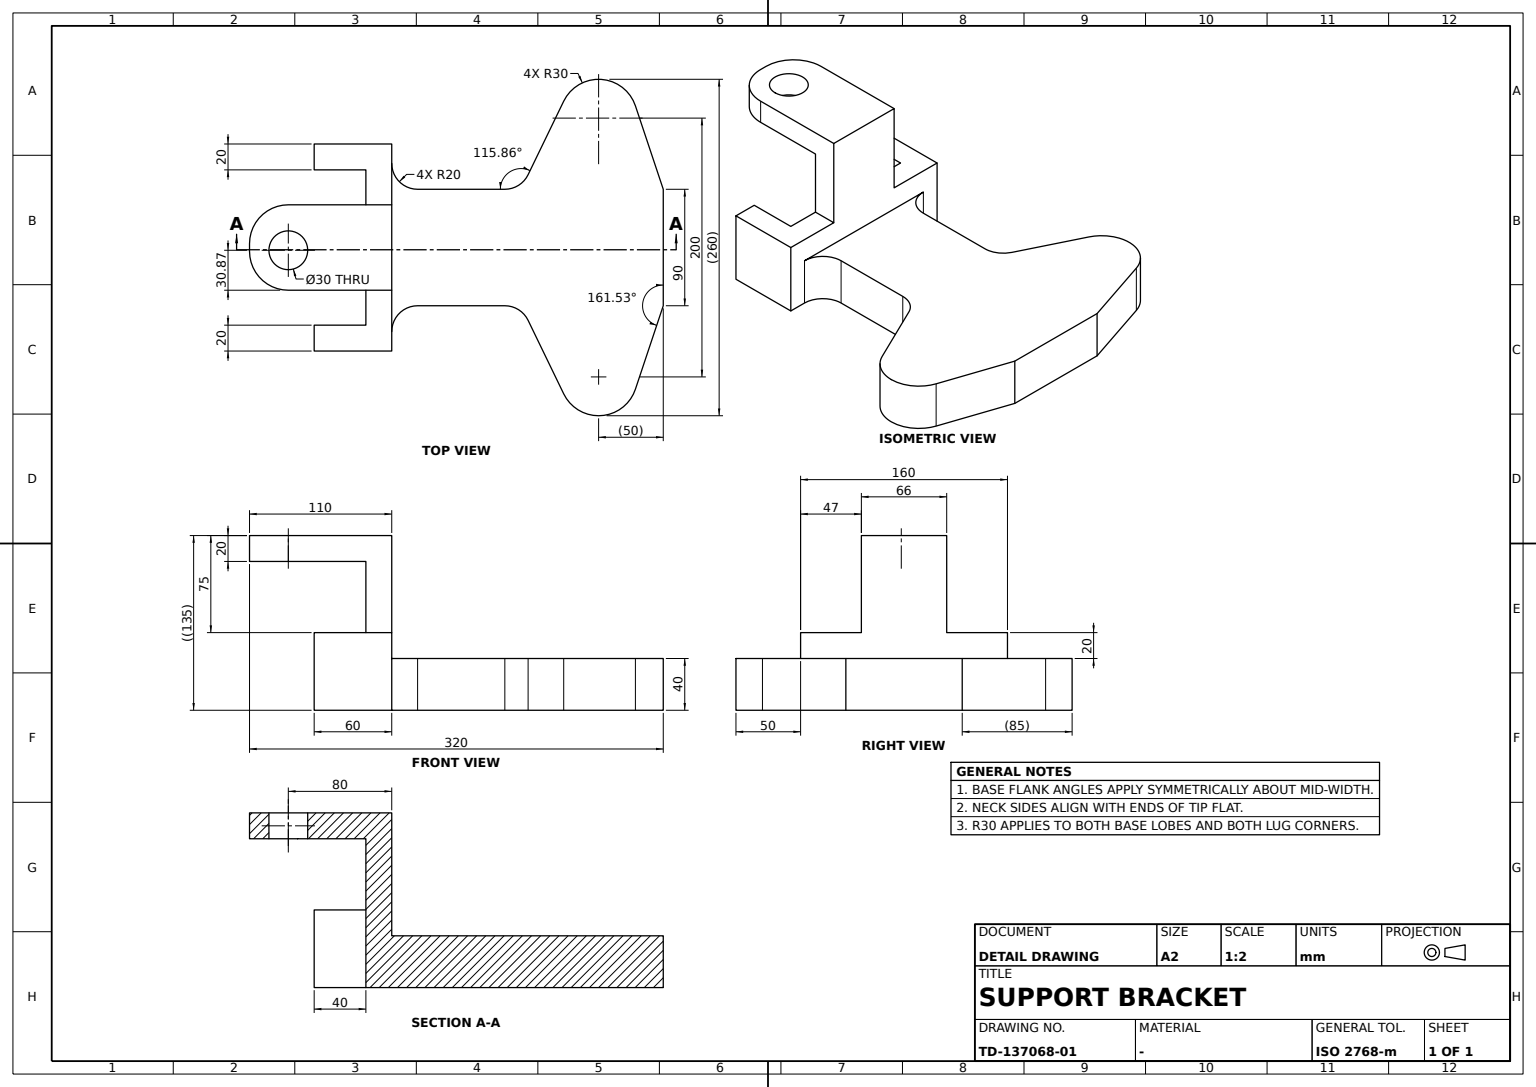
ISO-10303-21;
HEADER;
FILE_DESCRIPTION((''),'2;1');
FILE_NAME('','',(''),(''),'','','');
FILE_SCHEMA(('AUTOMOTIVE_DESIGN'));
ENDSEC;
DATA;
#1=APPLICATION_CONTEXT('');
#2=PRODUCT_CONTEXT('',#1,'mechanical');
#3=PRODUCT('','','',(#2));
#4=PRODUCT_DEFINITION_FORMATION('','',#3);
#5=PRODUCT_DEFINITION_CONTEXT('',#1,'design');
#6=PRODUCT_DEFINITION('','',#4,#5);
#7=PRODUCT_DEFINITION_SHAPE('','',#6);
#8=(LENGTH_UNIT()NAMED_UNIT(*)SI_UNIT(.MILLI.,.METRE.));
#9=(NAMED_UNIT(*)PLANE_ANGLE_UNIT()SI_UNIT($,.RADIAN.));
#10=(NAMED_UNIT(*)SI_UNIT($,.STERADIAN.)SOLID_ANGLE_UNIT());
#11=UNCERTAINTY_MEASURE_WITH_UNIT(LENGTH_MEASURE(1.E-05),#8,'distance_accuracy_value','');
#12=(GEOMETRIC_REPRESENTATION_CONTEXT(3)GLOBAL_UNCERTAINTY_ASSIGNED_CONTEXT((#11))GLOBAL_UNIT_ASSIGNED_CONTEXT((#8,#9,#10))REPRESENTATION_CONTEXT('',''));
#13=CARTESIAN_POINT('',(-80.,-220.,0.));
#14=VERTEX_POINT('',#13);
#15=CARTESIAN_POINT('',(-80.,-220.,60.));
#16=VERTEX_POINT('',#15);
#17=CARTESIAN_POINT('',(-80.,-220.,30.));
#18=DIRECTION('',(0.,0.,1.));
#19=VECTOR('',#18,1000.);
#20=LINE('',#17,#19);
#21=EDGE_CURVE('',#14,#16,#20,.T.);
#22=ORIENTED_EDGE('',*,*,#21,.T.);
#23=CARTESIAN_POINT('',(-80.,-160.,60.));
#24=VERTEX_POINT('',#23);
#25=CARTESIAN_POINT('',(-80.,-190.,60.));
#26=DIRECTION('',(0.,1.,0.));
#27=VECTOR('',#26,1000.);
#28=LINE('',#25,#27);
#29=EDGE_CURVE('',#16,#24,#28,.T.);
#30=ORIENTED_EDGE('',*,*,#29,.T.);
#31=CARTESIAN_POINT('',(-80.,-160.,0.));
#32=VERTEX_POINT('',#31);
#33=CARTESIAN_POINT('',(-80.,-160.,30.));
#34=LINE('',#33,#19);
#35=EDGE_CURVE('',#32,#24,#34,.T.);
#36=ORIENTED_EDGE('',*,*,#35,.F.);
#37=CARTESIAN_POINT('',(-80.,-190.,0.));
#38=LINE('',#37,#27);
#39=EDGE_CURVE('',#14,#32,#38,.T.);
#40=ORIENTED_EDGE('',*,*,#39,.F.);
#41=EDGE_LOOP('',(#22,#30,#36,#40));
#42=FACE_OUTER_BOUND('',#41,.T.);
#43=DIRECTION('',(-1.,0.,0.));
#44=DIRECTION('',(0.,-1.,0.));
#45=AXIS2_PLACEMENT_3D('',#31,#43,#44);
#46=PLANE('',#45);
#47=ADVANCED_FACE('',(#42),#46,.T.);
#48=CARTESIAN_POINT('',(33.,-240.,135.));
#49=VERTEX_POINT('',#48);
#50=CARTESIAN_POINT('',(33.,-240.,115.));
#51=VERTEX_POINT('',#50);
#52=CARTESIAN_POINT('',(33.,-240.,125.));
#53=DIRECTION('',(0.,0.,-1.));
#54=VECTOR('',#53,1000.);
#55=LINE('',#52,#54);
#56=EDGE_CURVE('',#49,#51,#55,.T.);
#57=ORIENTED_EDGE('',*,*,#56,.F.);
#58=CARTESIAN_POINT('',(3.,-270.,135.));
#59=VERTEX_POINT('',#58);
#60=CARTESIAN_POINT('',(3.,-240.,135.));
#61=AXIS2_PLACEMENT_3D('',#60,#53,#44);
#62=CIRCLE('',#61,30.);
#63=EDGE_CURVE('',#49,#59,#62,.T.);
#64=ORIENTED_EDGE('',*,*,#63,.T.);
#65=CARTESIAN_POINT('',(3.,-270.,115.));
#66=VERTEX_POINT('',#65);
#67=CARTESIAN_POINT('',(3.,-270.,125.));
#68=LINE('',#67,#54);
#69=EDGE_CURVE('',#59,#66,#68,.T.);
#70=ORIENTED_EDGE('',*,*,#69,.T.);
#71=CARTESIAN_POINT('',(3.,-240.,115.));
#72=AXIS2_PLACEMENT_3D('',#71,#18,#44);
#73=CIRCLE('',#72,30.);
#74=EDGE_CURVE('',#66,#51,#73,.T.);
#75=ORIENTED_EDGE('',*,*,#74,.T.);
#76=EDGE_LOOP('',(#57,#64,#70,#75));
#77=FACE_OUTER_BOUND('',#76,.T.);
#78=CARTESIAN_POINT('',(3.,-240.,97.5));
#79=AXIS2_PLACEMENT_3D('',#78,#18,#44);
#80=CYLINDRICAL_SURFACE('',#79,30.);
#81=ADVANCED_FACE('',(#77),#80,.T.);
#82=CARTESIAN_POINT('',(-56.276004,-54.533987,0.));
#83=VERTEX_POINT('',#82);
#84=CARTESIAN_POINT('',(-45.,-72.530984,0.));
#85=VERTEX_POINT('',#84);
#86=CARTESIAN_POINT('',(-65.,-72.530984,0.));
#87=DIRECTION('',(1.,0.,0.));
#88=AXIS2_PLACEMENT_3D('',#86,#53,#87);
#89=CIRCLE('',#88,20.);
#90=EDGE_CURVE('',#83,#85,#89,.T.);
#91=ORIENTED_EDGE('',*,*,#90,.T.);
#92=CARTESIAN_POINT('',(-45.,-72.530984,40.));
#93=VERTEX_POINT('',#92);
#94=CARTESIAN_POINT('',(-45.,-72.530984,20.));
#95=LINE('',#94,#19);
#96=EDGE_CURVE('',#85,#93,#95,.T.);
#97=ORIENTED_EDGE('',*,*,#96,.T.);
#98=CARTESIAN_POINT('',(-56.276004,-54.533987,40.));
#99=VERTEX_POINT('',#98);
#100=CARTESIAN_POINT('',(-65.,-72.530984,40.));
#101=AXIS2_PLACEMENT_3D('',#100,#53,#87);
#102=CIRCLE('',#101,20.);
#103=EDGE_CURVE('',#99,#93,#102,.T.);
#104=ORIENTED_EDGE('',*,*,#103,.F.);
#105=CARTESIAN_POINT('',(-56.276004,-54.533987,20.));
#106=LINE('',#105,#19);
#107=EDGE_CURVE('',#83,#99,#106,.T.);
#108=ORIENTED_EDGE('',*,*,#107,.F.);
#109=EDGE_LOOP('',(#91,#97,#104,#108));
#110=FACE_OUTER_BOUND('',#109,.T.);
#111=CARTESIAN_POINT('',(-65.,-72.530984,10.));
#112=AXIS2_PLACEMENT_3D('',#111,#53,#87);
#113=CYLINDRICAL_SURFACE('',#112,20.);
#114=ADVANCED_FACE('',(#110),#113,.F.);
#115=CARTESIAN_POINT('',(-109.504259,28.454684,0.));
#116=VERTEX_POINT('',#115);
#117=CARTESIAN_POINT('',(-109.504259,28.454684,40.));
#118=VERTEX_POINT('',#117);
#119=CARTESIAN_POINT('',(-109.504259,28.454684,20.));
#120=LINE('',#119,#19);
#121=EDGE_CURVE('',#116,#118,#120,.T.);
#122=ORIENTED_EDGE('',*,*,#121,.F.);
#123=CARTESIAN_POINT('',(-113.085994,-26.995495,0.));
#124=VERTEX_POINT('',#123);
#125=CARTESIAN_POINT('',(-100.,0.,0.));
#126=AXIS2_PLACEMENT_3D('',#125,#18,#87);
#127=CIRCLE('',#126,30.);
#128=EDGE_CURVE('',#116,#124,#127,.T.);
#129=ORIENTED_EDGE('',*,*,#128,.T.);
#130=CARTESIAN_POINT('',(-113.085994,-26.995495,40.));
#131=VERTEX_POINT('',#130);
#132=CARTESIAN_POINT('',(-113.085994,-26.995495,20.));
#133=LINE('',#132,#19);
#134=EDGE_CURVE('',#124,#131,#133,.T.);
#135=ORIENTED_EDGE('',*,*,#134,.T.);
#136=CARTESIAN_POINT('',(-100.,0.,40.));
#137=AXIS2_PLACEMENT_3D('',#136,#18,#87);
#138=CIRCLE('',#137,30.);
#139=EDGE_CURVE('',#118,#131,#138,.T.);
#140=ORIENTED_EDGE('',*,*,#139,.F.);
#141=EDGE_LOOP('',(#122,#129,#135,#140));
#142=FACE_OUTER_BOUND('',#141,.T.);
#143=CARTESIAN_POINT('',(-100.,0.,10.));
#144=AXIS2_PLACEMENT_3D('',#143,#53,#87);
#145=CYLINDRICAL_SURFACE('',#144,30.);
#146=ADVANCED_FACE('',(#142),#145,.T.);
#147=CARTESIAN_POINT('',(-33.,-160.,60.));
#148=VERTEX_POINT('',#147);
#149=CARTESIAN_POINT('',(-56.5,-160.,60.));
#150=VECTOR('',#87,1000.);
#151=LINE('',#149,#150);
#152=EDGE_CURVE('',#24,#148,#151,.T.);
#153=ORIENTED_EDGE('',*,*,#152,.F.);
#154=ORIENTED_EDGE('',*,*,#29,.F.);
#155=CARTESIAN_POINT('',(-60.,-220.,60.));
#156=VERTEX_POINT('',#155);
#157=CARTESIAN_POINT('',(-70.,-220.,60.));
#158=VECTOR('',#43,1000.);
#159=LINE('',#157,#158);
#160=EDGE_CURVE('',#156,#16,#159,.T.);
#161=ORIENTED_EDGE('',*,*,#160,.F.);
#162=CARTESIAN_POINT('',(-60.,-180.,60.));
#163=VERTEX_POINT('',#162);
#164=CARTESIAN_POINT('',(-60.,-200.,60.));
#165=VECTOR('',#44,1000.);
#166=LINE('',#164,#165);
#167=EDGE_CURVE('',#163,#156,#166,.T.);
#168=ORIENTED_EDGE('',*,*,#167,.F.);
#169=CARTESIAN_POINT('',(-33.,-180.,60.));
#170=VERTEX_POINT('',#169);
#171=CARTESIAN_POINT('',(-46.5,-180.,60.));
#172=LINE('',#171,#158);
#173=EDGE_CURVE('',#170,#163,#172,.T.);
#174=ORIENTED_EDGE('',*,*,#173,.F.);
#175=CARTESIAN_POINT('',(-33.,-170.,60.));
#176=LINE('',#175,#27);
#177=EDGE_CURVE('',#170,#148,#176,.T.);
#178=ORIENTED_EDGE('',*,*,#177,.T.);
#179=EDGE_LOOP('',(#153,#154,#161,#168,#174,#178));
#180=FACE_OUTER_BOUND('',#179,.T.);
#181=CARTESIAN_POINT('',(0.,0.,60.));
#182=AXIS2_PLACEMENT_3D('',#181,#53,#87);
#183=PLANE('',#182);
#184=ADVANCED_FACE('',(#180),#183,.F.);
#185=CARTESIAN_POINT('',(45.,50.,40.));
#186=VERTEX_POINT('',#185);
#187=CARTESIAN_POINT('',(-45.,50.,40.));
#188=VERTEX_POINT('',#187);
#189=CARTESIAN_POINT('',(0.,50.,40.));
#190=LINE('',#189,#158);
#191=EDGE_CURVE('',#186,#188,#190,.T.);
#192=ORIENTED_EDGE('',*,*,#191,.F.);
#193=CARTESIAN_POINT('',(45.,50.,0.));
#194=VERTEX_POINT('',#193);
#195=CARTESIAN_POINT('',(45.,50.,20.));
#196=LINE('',#195,#19);
#197=EDGE_CURVE('',#194,#186,#196,.T.);
#198=ORIENTED_EDGE('',*,*,#197,.F.);
#199=CARTESIAN_POINT('',(-45.,50.,0.));
#200=VERTEX_POINT('',#199);
#201=CARTESIAN_POINT('',(0.,50.,0.));
#202=LINE('',#201,#158);
#203=EDGE_CURVE('',#194,#200,#202,.T.);
#204=ORIENTED_EDGE('',*,*,#203,.T.);
#205=CARTESIAN_POINT('',(-45.,50.,20.));
#206=LINE('',#205,#19);
#207=EDGE_CURVE('',#200,#188,#206,.T.);
#208=ORIENTED_EDGE('',*,*,#207,.T.);
#209=EDGE_LOOP('',(#192,#198,#204,#208));
#210=FACE_OUTER_BOUND('',#209,.T.);
#211=AXIS2_PLACEMENT_3D('',#199,#44,#87);
#212=PLANE('',#211);
#213=ADVANCED_FACE('',(#210),#212,.F.);
#214=CARTESIAN_POINT('',(130.,0.,40.));
#215=VERTEX_POINT('',#214);
#216=CARTESIAN_POINT('',(109.504259,28.454684,40.));
#217=VERTEX_POINT('',#216);
#218=CARTESIAN_POINT('',(100.,0.,40.));
#219=AXIS2_PLACEMENT_3D('',#218,#18,#87);
#220=CIRCLE('',#219,30.);
#221=EDGE_CURVE('',#215,#217,#220,.T.);
#222=ORIENTED_EDGE('',*,*,#221,.F.);
#223=CARTESIAN_POINT('',(130.,0.,0.));
#224=VERTEX_POINT('',#223);
#225=CARTESIAN_POINT('',(130.,0.,10.));
#226=LINE('',#225,#54);
#227=EDGE_CURVE('',#215,#224,#226,.T.);
#228=ORIENTED_EDGE('',*,*,#227,.T.);
#229=CARTESIAN_POINT('',(109.504259,28.454684,0.));
#230=VERTEX_POINT('',#229);
#231=CARTESIAN_POINT('',(100.,0.,0.));
#232=AXIS2_PLACEMENT_3D('',#231,#18,#87);
#233=CIRCLE('',#232,30.);
#234=EDGE_CURVE('',#224,#230,#233,.T.);
#235=ORIENTED_EDGE('',*,*,#234,.T.);
#236=CARTESIAN_POINT('',(109.504259,28.454684,20.));
#237=LINE('',#236,#19);
#238=EDGE_CURVE('',#230,#217,#237,.T.);
#239=ORIENTED_EDGE('',*,*,#238,.T.);
#240=EDGE_LOOP('',(#222,#228,#235,#239));
#241=FACE_OUTER_BOUND('',#240,.T.);
#242=CARTESIAN_POINT('',(100.,0.,10.));
#243=AXIS2_PLACEMENT_3D('',#242,#53,#87);
#244=CYLINDRICAL_SURFACE('',#243,30.);
#245=ADVANCED_FACE('',(#241),#244,.T.);
#246=CARTESIAN_POINT('',(60.,-220.,60.));
#247=VERTEX_POINT('',#246);
#248=CARTESIAN_POINT('',(60.,-180.,60.));
#249=VERTEX_POINT('',#248);
#250=CARTESIAN_POINT('',(60.,-200.,60.));
#251=LINE('',#250,#27);
#252=EDGE_CURVE('',#247,#249,#251,.T.);
#253=ORIENTED_EDGE('',*,*,#252,.T.);
#254=CARTESIAN_POINT('',(60.,-180.,0.));
#255=VERTEX_POINT('',#254);
#256=CARTESIAN_POINT('',(60.,-180.,30.));
#257=LINE('',#256,#19);
#258=EDGE_CURVE('',#255,#249,#257,.T.);
#259=ORIENTED_EDGE('',*,*,#258,.F.);
#260=CARTESIAN_POINT('',(60.,-220.,0.));
#261=VERTEX_POINT('',#260);
#262=CARTESIAN_POINT('',(60.,-200.,0.));
#263=LINE('',#262,#27);
#264=EDGE_CURVE('',#261,#255,#263,.T.);
#265=ORIENTED_EDGE('',*,*,#264,.F.);
#266=CARTESIAN_POINT('',(60.,-220.,30.));
#267=LINE('',#266,#19);
#268=EDGE_CURVE('',#261,#247,#267,.T.);
#269=ORIENTED_EDGE('',*,*,#268,.T.);
#270=EDGE_LOOP('',(#253,#259,#265,#269));
#271=FACE_OUTER_BOUND('',#270,.T.);
#272=AXIS2_PLACEMENT_3D('',#254,#43,#44);
#273=PLANE('',#272);
#274=ADVANCED_FACE('',(#271),#273,.T.);
#275=CARTESIAN_POINT('',(15.289832,-247.191383,115.));
#276=VERTEX_POINT('',#275);
#277=CARTESIAN_POINT('',(15.289832,-247.191383,135.));
#278=VERTEX_POINT('',#277);
#279=CARTESIAN_POINT('',(15.289832,-247.191383,125.155));
#280=LINE('',#279,#19);
#281=EDGE_CURVE('',#276,#278,#280,.T.);
#282=ORIENTED_EDGE('',*,*,#281,.F.);
#283=CARTESIAN_POINT('',(-11.037645,-232.808617,115.));
#284=VERTEX_POINT('',#283);
#285=CARTESIAN_POINT('',(2.126093,-240.,115.));
#286=AXIS2_PLACEMENT_3D('',#285,#53,#87);
#287=CIRCLE('',#286,15.);
#288=EDGE_CURVE('',#276,#284,#287,.T.);
#289=ORIENTED_EDGE('',*,*,#288,.T.);
#290=CARTESIAN_POINT('',(-11.037645,-232.808617,135.));
#291=VERTEX_POINT('',#290);
#292=CARTESIAN_POINT('',(-11.037645,-232.808617,125.155));
#293=LINE('',#292,#19);
#294=EDGE_CURVE('',#284,#291,#293,.T.);
#295=ORIENTED_EDGE('',*,*,#294,.T.);
#296=CARTESIAN_POINT('',(2.126093,-240.,135.));
#297=AXIS2_PLACEMENT_3D('',#296,#18,#44);
#298=CIRCLE('',#297,15.);
#299=EDGE_CURVE('',#291,#278,#298,.T.);
#300=ORIENTED_EDGE('',*,*,#299,.T.);
#301=EDGE_LOOP('',(#282,#289,#295,#300));
#302=FACE_OUTER_BOUND('',#301,.T.);
#303=CARTESIAN_POINT('',(2.126093,-240.,134.9));
#304=AXIS2_PLACEMENT_3D('',#303,#18,#87);
#305=CYLINDRICAL_SURFACE('',#304,15.);
#306=ADVANCED_FACE('',(#302),#305,.F.);
#307=ORIENTED_EDGE('',*,*,#227,.F.);
#308=CARTESIAN_POINT('',(113.085994,-26.995495,40.));
#309=VERTEX_POINT('',#308);
#310=EDGE_CURVE('',#309,#215,#220,.T.);
#311=ORIENTED_EDGE('',*,*,#310,.F.);
#312=CARTESIAN_POINT('',(113.085994,-26.995495,0.));
#313=VERTEX_POINT('',#312);
#314=CARTESIAN_POINT('',(113.085994,-26.995495,20.));
#315=LINE('',#314,#19);
#316=EDGE_CURVE('',#313,#309,#315,.T.);
#317=ORIENTED_EDGE('',*,*,#316,.F.);
#318=EDGE_CURVE('',#313,#224,#233,.T.);
#319=ORIENTED_EDGE('',*,*,#318,.T.);
#320=EDGE_LOOP('',(#307,#311,#317,#319));
#321=FACE_OUTER_BOUND('',#320,.T.);
#322=ADVANCED_FACE('',(#321),#244,.T.);
#323=CARTESIAN_POINT('',(17.126093,-240.,135.));
#324=VERTEX_POINT('',#323);
#325=EDGE_CURVE('',#324,#291,#298,.T.);
#326=ORIENTED_EDGE('',*,*,#325,.T.);
#327=ORIENTED_EDGE('',*,*,#294,.F.);
#328=CARTESIAN_POINT('',(17.126093,-240.,115.));
#329=VERTEX_POINT('',#328);
#330=EDGE_CURVE('',#284,#329,#287,.T.);
#331=ORIENTED_EDGE('',*,*,#330,.T.);
#332=CARTESIAN_POINT('',(17.126093,-240.,134.9));
#333=LINE('',#332,#19);
#334=EDGE_CURVE('',#329,#324,#333,.T.);
#335=ORIENTED_EDGE('',*,*,#334,.T.);
#336=EDGE_LOOP('',(#326,#327,#331,#335));
#337=FACE_OUTER_BOUND('',#336,.T.);
#338=ADVANCED_FACE('',(#337),#305,.F.);
#339=CARTESIAN_POINT('',(-77.252129,39.227342,0.));
#340=DIRECTION('',(-0.948489482,-0.31680862,0.));
#341=VECTOR('',#340,1000.);
#342=LINE('',#339,#341);
#343=EDGE_CURVE('',#200,#116,#342,.T.);
#344=ORIENTED_EDGE('',*,*,#343,.T.);
#345=ORIENTED_EDGE('',*,*,#121,.T.);
#346=CARTESIAN_POINT('',(-77.252129,39.227342,40.));
#347=LINE('',#346,#341);
#348=EDGE_CURVE('',#188,#118,#347,.T.);
#349=ORIENTED_EDGE('',*,*,#348,.F.);
#350=ORIENTED_EDGE('',*,*,#207,.F.);
#351=EDGE_LOOP('',(#344,#345,#349,#350));
#352=FACE_OUTER_BOUND('',#351,.T.);
#353=DIRECTION('',(0.31680862,-0.948489482,0.));
#354=DIRECTION('',(0.948489482,0.31680862,0.));
#355=AXIS2_PLACEMENT_3D('',#115,#353,#354);
#356=PLANE('',#355);
#357=ADVANCED_FACE('',(#352),#356,.F.);
#358=CARTESIAN_POINT('',(-45.,-140.,0.));
#359=VERTEX_POINT('',#358);
#360=CARTESIAN_POINT('',(-65.,-160.,0.));
#361=VERTEX_POINT('',#360);
#362=CARTESIAN_POINT('',(-65.,-140.,0.));
#363=AXIS2_PLACEMENT_3D('',#362,#53,#87);
#364=CIRCLE('',#363,20.);
#365=EDGE_CURVE('',#359,#361,#364,.T.);
#366=ORIENTED_EDGE('',*,*,#365,.T.);
#367=CARTESIAN_POINT('',(-65.,-160.,40.));
#368=VERTEX_POINT('',#367);
#369=CARTESIAN_POINT('',(-65.,-160.,20.));
#370=LINE('',#369,#19);
#371=EDGE_CURVE('',#361,#368,#370,.T.);
#372=ORIENTED_EDGE('',*,*,#371,.T.);
#373=CARTESIAN_POINT('',(-45.,-140.,40.));
#374=VERTEX_POINT('',#373);
#375=CARTESIAN_POINT('',(-65.,-140.,40.));
#376=AXIS2_PLACEMENT_3D('',#375,#53,#87);
#377=CIRCLE('',#376,20.);
#378=EDGE_CURVE('',#374,#368,#377,.T.);
#379=ORIENTED_EDGE('',*,*,#378,.F.);
#380=CARTESIAN_POINT('',(-45.,-140.,20.));
#381=LINE('',#380,#19);
#382=EDGE_CURVE('',#359,#374,#381,.T.);
#383=ORIENTED_EDGE('',*,*,#382,.F.);
#384=EDGE_LOOP('',(#366,#372,#379,#383));
#385=FACE_OUTER_BOUND('',#384,.T.);
#386=CARTESIAN_POINT('',(-65.,-140.,10.));
#387=AXIS2_PLACEMENT_3D('',#386,#53,#87);
#388=CYLINDRICAL_SURFACE('',#387,20.);
#389=ADVANCED_FACE('',(#385),#388,.F.);
#390=ORIENTED_EDGE('',*,*,#268,.F.);
#391=CARTESIAN_POINT('',(80.,-220.,0.));
#392=VERTEX_POINT('',#391);
#393=CARTESIAN_POINT('',(70.,-220.,0.));
#394=LINE('',#393,#158);
#395=EDGE_CURVE('',#392,#261,#394,.T.);
#396=ORIENTED_EDGE('',*,*,#395,.F.);
#397=CARTESIAN_POINT('',(80.,-220.,60.));
#398=VERTEX_POINT('',#397);
#399=CARTESIAN_POINT('',(80.,-220.,30.));
#400=LINE('',#399,#19);
#401=EDGE_CURVE('',#392,#398,#400,.T.);
#402=ORIENTED_EDGE('',*,*,#401,.T.);
#403=CARTESIAN_POINT('',(70.,-220.,60.));
#404=LINE('',#403,#158);
#405=EDGE_CURVE('',#398,#247,#404,.T.);
#406=ORIENTED_EDGE('',*,*,#405,.T.);
#407=EDGE_LOOP('',(#390,#396,#402,#406));
#408=FACE_OUTER_BOUND('',#407,.T.);
#409=AXIS2_PLACEMENT_3D('',#391,#26,#43);
#410=PLANE('',#409);
#411=ADVANCED_FACE('',(#408),#410,.F.);
#412=CARTESIAN_POINT('',(-33.,-160.,135.));
#413=VERTEX_POINT('',#412);
#414=CARTESIAN_POINT('',(-33.,-240.,135.));
#415=VERTEX_POINT('',#414);
#416=CARTESIAN_POINT('',(-33.,-200.,135.));
#417=LINE('',#416,#165);
#418=EDGE_CURVE('',#413,#415,#417,.T.);
#419=ORIENTED_EDGE('',*,*,#418,.F.);
#420=CARTESIAN_POINT('',(-33.,-160.,97.5));
#421=LINE('',#420,#19);
#422=EDGE_CURVE('',#148,#413,#421,.T.);
#423=ORIENTED_EDGE('',*,*,#422,.F.);
#424=ORIENTED_EDGE('',*,*,#177,.F.);
#425=CARTESIAN_POINT('',(-33.,-180.,115.));
#426=VERTEX_POINT('',#425);
#427=CARTESIAN_POINT('',(-33.,-180.,87.5));
#428=LINE('',#427,#54);
#429=EDGE_CURVE('',#426,#170,#428,.T.);
#430=ORIENTED_EDGE('',*,*,#429,.F.);
#431=CARTESIAN_POINT('',(-33.,-240.,115.));
#432=VERTEX_POINT('',#431);
#433=CARTESIAN_POINT('',(-33.,-210.,115.));
#434=LINE('',#433,#27);
#435=EDGE_CURVE('',#432,#426,#434,.T.);
#436=ORIENTED_EDGE('',*,*,#435,.F.);
#437=CARTESIAN_POINT('',(-33.,-240.,125.));
#438=LINE('',#437,#54);
#439=EDGE_CURVE('',#415,#432,#438,.T.);
#440=ORIENTED_EDGE('',*,*,#439,.F.);
#441=EDGE_LOOP('',(#419,#423,#424,#430,#436,#440));
#442=FACE_OUTER_BOUND('',#441,.T.);
#443=CARTESIAN_POINT('',(-33.,0.,0.));
#444=AXIS2_PLACEMENT_3D('',#443,#87,#26);
#445=PLANE('',#444);
#446=ADVANCED_FACE('',(#442),#445,.F.);
#447=CARTESIAN_POINT('',(-3.,-270.,135.));
#448=VERTEX_POINT('',#447);
#449=CARTESIAN_POINT('',(-3.,-240.,135.));
#450=AXIS2_PLACEMENT_3D('',#449,#53,#44);
#451=CIRCLE('',#450,30.);
#452=EDGE_CURVE('',#448,#415,#451,.T.);
#453=ORIENTED_EDGE('',*,*,#452,.T.);
#454=ORIENTED_EDGE('',*,*,#439,.T.);
#455=CARTESIAN_POINT('',(-3.,-270.,115.));
#456=VERTEX_POINT('',#455);
#457=CARTESIAN_POINT('',(-3.,-240.,115.));
#458=AXIS2_PLACEMENT_3D('',#457,#18,#44);
#459=CIRCLE('',#458,30.);
#460=EDGE_CURVE('',#432,#456,#459,.T.);
#461=ORIENTED_EDGE('',*,*,#460,.T.);
#462=CARTESIAN_POINT('',(-3.,-270.,125.));
#463=LINE('',#462,#54);
#464=EDGE_CURVE('',#448,#456,#463,.T.);
#465=ORIENTED_EDGE('',*,*,#464,.F.);
#466=EDGE_LOOP('',(#453,#454,#461,#465));
#467=FACE_OUTER_BOUND('',#466,.T.);
#468=CARTESIAN_POINT('',(-3.,-240.,97.5));
#469=AXIS2_PLACEMENT_3D('',#468,#18,#43);
#470=CYLINDRICAL_SURFACE('',#469,30.);
#471=ADVANCED_FACE('',(#467),#470,.T.);
#472=ORIENTED_EDGE('',*,*,#371,.F.);
#473=CARTESIAN_POINT('',(-72.5,-160.,0.));
#474=LINE('',#473,#150);
#475=EDGE_CURVE('',#32,#361,#474,.T.);
#476=ORIENTED_EDGE('',*,*,#475,.F.);
#477=ORIENTED_EDGE('',*,*,#35,.T.);
#478=ORIENTED_EDGE('',*,*,#152,.T.);
#479=ORIENTED_EDGE('',*,*,#422,.T.);
#480=CARTESIAN_POINT('',(33.,-160.,135.));
#481=VERTEX_POINT('',#480);
#482=CARTESIAN_POINT('',(0.,-160.,135.));
#483=LINE('',#482,#150);
#484=EDGE_CURVE('',#413,#481,#483,.T.);
#485=ORIENTED_EDGE('',*,*,#484,.T.);
#486=CARTESIAN_POINT('',(33.,-160.,60.));
#487=VERTEX_POINT('',#486);
#488=CARTESIAN_POINT('',(33.,-160.,97.5));
#489=LINE('',#488,#19);
#490=EDGE_CURVE('',#487,#481,#489,.T.);
#491=ORIENTED_EDGE('',*,*,#490,.F.);
#492=CARTESIAN_POINT('',(80.,-160.,60.));
#493=VERTEX_POINT('',#492);
#494=CARTESIAN_POINT('',(56.5,-160.,60.));
#495=LINE('',#494,#150);
#496=EDGE_CURVE('',#487,#493,#495,.T.);
#497=ORIENTED_EDGE('',*,*,#496,.T.);
#498=CARTESIAN_POINT('',(80.,-160.,0.));
#499=VERTEX_POINT('',#498);
#500=CARTESIAN_POINT('',(80.,-160.,30.));
#501=LINE('',#500,#19);
#502=EDGE_CURVE('',#499,#493,#501,.T.);
#503=ORIENTED_EDGE('',*,*,#502,.F.);
#504=CARTESIAN_POINT('',(65.,-160.,0.));
#505=VERTEX_POINT('',#504);
#506=CARTESIAN_POINT('',(72.5,-160.,0.));
#507=LINE('',#506,#150);
#508=EDGE_CURVE('',#505,#499,#507,.T.);
#509=ORIENTED_EDGE('',*,*,#508,.F.);
#510=CARTESIAN_POINT('',(65.,-160.,40.));
#511=VERTEX_POINT('',#510);
#512=CARTESIAN_POINT('',(65.,-160.,20.));
#513=LINE('',#512,#19);
#514=EDGE_CURVE('',#505,#511,#513,.T.);
#515=ORIENTED_EDGE('',*,*,#514,.T.);
#516=CARTESIAN_POINT('',(0.,-160.,40.));
#517=LINE('',#516,#150);
#518=EDGE_CURVE('',#368,#511,#517,.T.);
#519=ORIENTED_EDGE('',*,*,#518,.F.);
#520=EDGE_LOOP('',(#472,#476,#477,#478,#479,#485,#491,#497,#503,#509,#515,#519));
#521=FACE_OUTER_BOUND('',#520,.T.);
#522=AXIS2_PLACEMENT_3D('',#360,#44,#87);
#523=PLANE('',#522);
#524=ADVANCED_FACE('',(#521),#523,.F.);
#525=CARTESIAN_POINT('',(-84.680999,-40.764741,40.));
#526=DIRECTION('',(0.899849832,-0.436199817,0.));
#527=VECTOR('',#526,1000.);
#528=LINE('',#525,#527);
#529=EDGE_CURVE('',#131,#99,#528,.T.);
#530=ORIENTED_EDGE('',*,*,#529,.F.);
#531=ORIENTED_EDGE('',*,*,#134,.F.);
#532=CARTESIAN_POINT('',(-84.680999,-40.764741,0.));
#533=LINE('',#532,#527);
#534=EDGE_CURVE('',#124,#83,#533,.T.);
#535=ORIENTED_EDGE('',*,*,#534,.T.);
#536=ORIENTED_EDGE('',*,*,#107,.T.);
#537=EDGE_LOOP('',(#530,#531,#535,#536));
#538=FACE_OUTER_BOUND('',#537,.T.);
#539=DIRECTION('',(0.436199817,0.899849832,0.));
#540=DIRECTION('',(-0.899849832,0.436199817,0.));
#541=AXIS2_PLACEMENT_3D('',#82,#539,#540);
#542=PLANE('',#541);
#543=ADVANCED_FACE('',(#538),#542,.F.);
#544=ORIENTED_EDGE('',*,*,#197,.T.);
#545=CARTESIAN_POINT('',(77.252129,39.227342,40.));
#546=DIRECTION('',(-0.948489482,0.31680862,0.));
#547=VECTOR('',#546,1000.);
#548=LINE('',#545,#547);
#549=EDGE_CURVE('',#217,#186,#548,.T.);
#550=ORIENTED_EDGE('',*,*,#549,.F.);
#551=ORIENTED_EDGE('',*,*,#238,.F.);
#552=CARTESIAN_POINT('',(77.252129,39.227342,0.));
#553=LINE('',#552,#547);
#554=EDGE_CURVE('',#230,#194,#553,.T.);
#555=ORIENTED_EDGE('',*,*,#554,.T.);
#556=EDGE_LOOP('',(#544,#550,#551,#555));
#557=FACE_OUTER_BOUND('',#556,.T.);
#558=DIRECTION('',(0.31680862,0.948489482,0.));
#559=AXIS2_PLACEMENT_3D('',#229,#558,#546);
#560=PLANE('',#559);
#561=ADVANCED_FACE('',(#557),#560,.T.);
#562=CARTESIAN_POINT('',(45.,-72.530984,40.));
#563=VERTEX_POINT('',#562);
#564=CARTESIAN_POINT('',(56.276004,-54.533987,40.));
#565=VERTEX_POINT('',#564);
#566=CARTESIAN_POINT('',(65.,-72.530984,40.));
#567=AXIS2_PLACEMENT_3D('',#566,#53,#87);
#568=CIRCLE('',#567,20.);
#569=EDGE_CURVE('',#563,#565,#568,.T.);
#570=ORIENTED_EDGE('',*,*,#569,.F.);
#571=CARTESIAN_POINT('',(45.,-72.530984,0.));
#572=VERTEX_POINT('',#571);
#573=CARTESIAN_POINT('',(45.,-72.530984,20.));
#574=LINE('',#573,#19);
#575=EDGE_CURVE('',#572,#563,#574,.T.);
#576=ORIENTED_EDGE('',*,*,#575,.F.);
#577=CARTESIAN_POINT('',(56.276004,-54.533987,0.));
#578=VERTEX_POINT('',#577);
#579=CARTESIAN_POINT('',(65.,-72.530984,0.));
#580=AXIS2_PLACEMENT_3D('',#579,#53,#87);
#581=CIRCLE('',#580,20.);
#582=EDGE_CURVE('',#572,#578,#581,.T.);
#583=ORIENTED_EDGE('',*,*,#582,.T.);
#584=CARTESIAN_POINT('',(56.276004,-54.533987,20.));
#585=LINE('',#584,#19);
#586=EDGE_CURVE('',#578,#565,#585,.T.);
#587=ORIENTED_EDGE('',*,*,#586,.T.);
#588=EDGE_LOOP('',(#570,#576,#583,#587));
#589=FACE_OUTER_BOUND('',#588,.T.);
#590=CARTESIAN_POINT('',(65.,-72.530984,10.));
#591=AXIS2_PLACEMENT_3D('',#590,#53,#87);
#592=CYLINDRICAL_SURFACE('',#591,20.);
#593=ADVANCED_FACE('',(#589),#592,.F.);
#594=CARTESIAN_POINT('',(45.,-140.,40.));
#595=VERTEX_POINT('',#594);
#596=CARTESIAN_POINT('',(45.,-106.265492,40.));
#597=LINE('',#596,#27);
#598=EDGE_CURVE('',#595,#563,#597,.T.);
#599=ORIENTED_EDGE('',*,*,#598,.F.);
#600=CARTESIAN_POINT('',(45.,-140.,0.));
#601=VERTEX_POINT('',#600);
#602=CARTESIAN_POINT('',(45.,-140.,20.));
#603=LINE('',#602,#19);
#604=EDGE_CURVE('',#601,#595,#603,.T.);
#605=ORIENTED_EDGE('',*,*,#604,.F.);
#606=CARTESIAN_POINT('',(45.,-106.265492,0.));
#607=LINE('',#606,#27);
#608=EDGE_CURVE('',#601,#572,#607,.T.);
#609=ORIENTED_EDGE('',*,*,#608,.T.);
#610=ORIENTED_EDGE('',*,*,#575,.T.);
#611=EDGE_LOOP('',(#599,#605,#609,#610));
#612=FACE_OUTER_BOUND('',#611,.T.);
#613=AXIS2_PLACEMENT_3D('',#571,#43,#44);
#614=PLANE('',#613);
#615=ADVANCED_FACE('',(#612),#614,.F.);
#616=ORIENTED_EDGE('',*,*,#401,.F.);
#617=CARTESIAN_POINT('',(80.,-190.,0.));
#618=LINE('',#617,#165);
#619=EDGE_CURVE('',#499,#392,#618,.T.);
#620=ORIENTED_EDGE('',*,*,#619,.F.);
#621=ORIENTED_EDGE('',*,*,#502,.T.);
#622=CARTESIAN_POINT('',(80.,-190.,60.));
#623=LINE('',#622,#165);
#624=EDGE_CURVE('',#493,#398,#623,.T.);
#625=ORIENTED_EDGE('',*,*,#624,.T.);
#626=EDGE_LOOP('',(#616,#620,#621,#625));
#627=FACE_OUTER_BOUND('',#626,.T.);
#628=AXIS2_PLACEMENT_3D('',#498,#43,#44);
#629=PLANE('',#628);
#630=ADVANCED_FACE('',(#627),#629,.F.);
#631=ORIENTED_EDGE('',*,*,#173,.T.);
#632=CARTESIAN_POINT('',(-60.,-180.,0.));
#633=VERTEX_POINT('',#632);
#634=CARTESIAN_POINT('',(-60.,-180.,30.));
#635=LINE('',#634,#19);
#636=EDGE_CURVE('',#633,#163,#635,.T.);
#637=ORIENTED_EDGE('',*,*,#636,.F.);
#638=CARTESIAN_POINT('',(0.,-180.,0.));
#639=LINE('',#638,#158);
#640=EDGE_CURVE('',#255,#633,#639,.T.);
#641=ORIENTED_EDGE('',*,*,#640,.F.);
#642=ORIENTED_EDGE('',*,*,#258,.T.);
#643=CARTESIAN_POINT('',(33.,-180.,60.));
#644=VERTEX_POINT('',#643);
#645=CARTESIAN_POINT('',(46.5,-180.,60.));
#646=LINE('',#645,#158);
#647=EDGE_CURVE('',#249,#644,#646,.T.);
#648=ORIENTED_EDGE('',*,*,#647,.T.);
#649=CARTESIAN_POINT('',(33.,-180.,115.));
#650=VERTEX_POINT('',#649);
#651=CARTESIAN_POINT('',(33.,-180.,87.5));
#652=LINE('',#651,#54);
#653=EDGE_CURVE('',#650,#644,#652,.T.);
#654=ORIENTED_EDGE('',*,*,#653,.F.);
#655=CARTESIAN_POINT('',(0.,-180.,115.));
#656=LINE('',#655,#150);
#657=EDGE_CURVE('',#426,#650,#656,.T.);
#658=ORIENTED_EDGE('',*,*,#657,.F.);
#659=ORIENTED_EDGE('',*,*,#429,.T.);
#660=EDGE_LOOP('',(#631,#637,#641,#642,#648,#654,#658,#659));
#661=FACE_OUTER_BOUND('',#660,.T.);
#662=AXIS2_PLACEMENT_3D('',#632,#44,#87);
#663=PLANE('',#662);
#664=ADVANCED_FACE('',(#661),#663,.T.);
#665=ORIENTED_EDGE('',*,*,#330,.F.);
#666=ORIENTED_EDGE('',*,*,#288,.F.);
#667=EDGE_CURVE('',#329,#276,#287,.T.);
#668=ORIENTED_EDGE('',*,*,#667,.F.);
#669=EDGE_LOOP('',(#665,#666,#668));
#670=FACE_BOUND('',#669,.T.);
#671=ORIENTED_EDGE('',*,*,#460,.F.);
#672=ORIENTED_EDGE('',*,*,#435,.T.);
#673=ORIENTED_EDGE('',*,*,#657,.T.);
#674=CARTESIAN_POINT('',(33.,-210.,115.));
#675=LINE('',#674,#27);
#676=EDGE_CURVE('',#51,#650,#675,.T.);
#677=ORIENTED_EDGE('',*,*,#676,.F.);
#678=ORIENTED_EDGE('',*,*,#74,.F.);
#679=CARTESIAN_POINT('',(0.,-270.,115.));
#680=LINE('',#679,#150);
#681=EDGE_CURVE('',#456,#66,#680,.T.);
#682=ORIENTED_EDGE('',*,*,#681,.F.);
#683=EDGE_LOOP('',(#671,#672,#673,#677,#678,#682));
#684=FACE_OUTER_BOUND('',#683,.T.);
#685=AXIS2_PLACEMENT_3D('',#655,#18,#44);
#686=PLANE('',#685);
#687=ADVANCED_FACE('',(#670,#684),#686,.F.);
#688=ORIENTED_EDGE('',*,*,#382,.T.);
#689=CARTESIAN_POINT('',(-45.,-106.265492,40.));
#690=LINE('',#689,#165);
#691=EDGE_CURVE('',#93,#374,#690,.T.);
#692=ORIENTED_EDGE('',*,*,#691,.F.);
#693=ORIENTED_EDGE('',*,*,#96,.F.);
#694=CARTESIAN_POINT('',(-45.,-106.265492,0.));
#695=LINE('',#694,#165);
#696=EDGE_CURVE('',#85,#359,#695,.T.);
#697=ORIENTED_EDGE('',*,*,#696,.T.);
#698=EDGE_LOOP('',(#688,#692,#693,#697));
#699=FACE_OUTER_BOUND('',#698,.T.);
#700=AXIS2_PLACEMENT_3D('',#84,#43,#44);
#701=PLANE('',#700);
#702=ADVANCED_FACE('',(#699),#701,.T.);
#703=ORIENTED_EDGE('',*,*,#667,.T.);
#704=ORIENTED_EDGE('',*,*,#281,.T.);
#705=EDGE_CURVE('',#278,#324,#298,.T.);
#706=ORIENTED_EDGE('',*,*,#705,.T.);
#707=ORIENTED_EDGE('',*,*,#334,.F.);
#708=EDGE_LOOP('',(#703,#704,#706,#707));
#709=FACE_OUTER_BOUND('',#708,.T.);
#710=ADVANCED_FACE('',(#709),#305,.F.);
#711=ORIENTED_EDGE('',*,*,#299,.F.);
#712=ORIENTED_EDGE('',*,*,#325,.F.);
#713=ORIENTED_EDGE('',*,*,#705,.F.);
#714=EDGE_LOOP('',(#711,#712,#713));
#715=FACE_BOUND('',#714,.T.);
#716=ORIENTED_EDGE('',*,*,#418,.T.);
#717=ORIENTED_EDGE('',*,*,#452,.F.);
#718=CARTESIAN_POINT('',(0.,-270.,135.));
#719=LINE('',#718,#150);
#720=EDGE_CURVE('',#448,#59,#719,.T.);
#721=ORIENTED_EDGE('',*,*,#720,.T.);
#722=ORIENTED_EDGE('',*,*,#63,.F.);
#723=CARTESIAN_POINT('',(33.,-200.,135.));
#724=LINE('',#723,#165);
#725=EDGE_CURVE('',#481,#49,#724,.T.);
#726=ORIENTED_EDGE('',*,*,#725,.F.);
#727=ORIENTED_EDGE('',*,*,#484,.F.);
#728=EDGE_LOOP('',(#716,#717,#721,#722,#726,#727));
#729=FACE_OUTER_BOUND('',#728,.T.);
#730=AXIS2_PLACEMENT_3D('',#482,#18,#44);
#731=PLANE('',#730);
#732=ADVANCED_FACE('',(#715,#729),#731,.T.);
#733=ORIENTED_EDGE('',*,*,#647,.F.);
#734=ORIENTED_EDGE('',*,*,#252,.F.);
#735=ORIENTED_EDGE('',*,*,#405,.F.);
#736=ORIENTED_EDGE('',*,*,#624,.F.);
#737=ORIENTED_EDGE('',*,*,#496,.F.);
#738=CARTESIAN_POINT('',(33.,-170.,60.));
#739=LINE('',#738,#27);
#740=EDGE_CURVE('',#644,#487,#739,.T.);
#741=ORIENTED_EDGE('',*,*,#740,.F.);
#742=EDGE_LOOP('',(#733,#734,#735,#736,#737,#741));
#743=FACE_OUTER_BOUND('',#742,.T.);
#744=ADVANCED_FACE('',(#743),#183,.F.);
#745=ORIENTED_EDGE('',*,*,#676,.T.);
#746=ORIENTED_EDGE('',*,*,#653,.T.);
#747=ORIENTED_EDGE('',*,*,#740,.T.);
#748=ORIENTED_EDGE('',*,*,#490,.T.);
#749=ORIENTED_EDGE('',*,*,#725,.T.);
#750=ORIENTED_EDGE('',*,*,#56,.T.);
#751=EDGE_LOOP('',(#745,#746,#747,#748,#749,#750));
#752=FACE_OUTER_BOUND('',#751,.T.);
#753=CARTESIAN_POINT('',(33.,0.,0.));
#754=AXIS2_PLACEMENT_3D('',#753,#87,#26);
#755=PLANE('',#754);
#756=ADVANCED_FACE('',(#752),#755,.T.);
#757=ORIENTED_EDGE('',*,*,#691,.T.);
#758=ORIENTED_EDGE('',*,*,#378,.T.);
#759=ORIENTED_EDGE('',*,*,#518,.T.);
#760=CARTESIAN_POINT('',(65.,-140.,40.));
#761=AXIS2_PLACEMENT_3D('',#760,#53,#87);
#762=CIRCLE('',#761,20.);
#763=EDGE_CURVE('',#511,#595,#762,.T.);
#764=ORIENTED_EDGE('',*,*,#763,.T.);
#765=ORIENTED_EDGE('',*,*,#598,.T.);
#766=ORIENTED_EDGE('',*,*,#569,.T.);
#767=CARTESIAN_POINT('',(84.680999,-40.764741,40.));
#768=DIRECTION('',(0.899849832,0.436199817,0.));
#769=VECTOR('',#768,1000.);
#770=LINE('',#767,#769);
#771=EDGE_CURVE('',#565,#309,#770,.T.);
#772=ORIENTED_EDGE('',*,*,#771,.T.);
#773=ORIENTED_EDGE('',*,*,#310,.T.);
#774=ORIENTED_EDGE('',*,*,#221,.T.);
#775=ORIENTED_EDGE('',*,*,#549,.T.);
#776=ORIENTED_EDGE('',*,*,#191,.T.);
#777=ORIENTED_EDGE('',*,*,#348,.T.);
#778=ORIENTED_EDGE('',*,*,#139,.T.);
#779=ORIENTED_EDGE('',*,*,#529,.T.);
#780=ORIENTED_EDGE('',*,*,#103,.T.);
#781=EDGE_LOOP('',(#757,#758,#759,#764,#765,#766,#772,#773,#774,#775,#776,#777,#778,#779,#780));
#782=FACE_OUTER_BOUND('',#781,.T.);
#783=CARTESIAN_POINT('',(0.,0.,40.));
#784=AXIS2_PLACEMENT_3D('',#783,#18,#87);
#785=PLANE('',#784);
#786=ADVANCED_FACE('',(#782),#785,.T.);
#787=ORIENTED_EDGE('',*,*,#508,.T.);
#788=ORIENTED_EDGE('',*,*,#619,.T.);
#789=ORIENTED_EDGE('',*,*,#395,.T.);
#790=ORIENTED_EDGE('',*,*,#264,.T.);
#791=ORIENTED_EDGE('',*,*,#640,.T.);
#792=CARTESIAN_POINT('',(-60.,-220.,0.));
#793=VERTEX_POINT('',#792);
#794=CARTESIAN_POINT('',(-60.,-200.,0.));
#795=LINE('',#794,#165);
#796=EDGE_CURVE('',#633,#793,#795,.T.);
#797=ORIENTED_EDGE('',*,*,#796,.T.);
#798=CARTESIAN_POINT('',(-70.,-220.,0.));
#799=LINE('',#798,#158);
#800=EDGE_CURVE('',#793,#14,#799,.T.);
#801=ORIENTED_EDGE('',*,*,#800,.T.);
#802=ORIENTED_EDGE('',*,*,#39,.T.);
#803=ORIENTED_EDGE('',*,*,#475,.T.);
#804=ORIENTED_EDGE('',*,*,#365,.F.);
#805=ORIENTED_EDGE('',*,*,#696,.F.);
#806=ORIENTED_EDGE('',*,*,#90,.F.);
#807=ORIENTED_EDGE('',*,*,#534,.F.);
#808=ORIENTED_EDGE('',*,*,#128,.F.);
#809=ORIENTED_EDGE('',*,*,#343,.F.);
#810=ORIENTED_EDGE('',*,*,#203,.F.);
#811=ORIENTED_EDGE('',*,*,#554,.F.);
#812=ORIENTED_EDGE('',*,*,#234,.F.);
#813=ORIENTED_EDGE('',*,*,#318,.F.);
#814=CARTESIAN_POINT('',(84.680999,-40.764741,0.));
#815=LINE('',#814,#769);
#816=EDGE_CURVE('',#578,#313,#815,.T.);
#817=ORIENTED_EDGE('',*,*,#816,.F.);
#818=ORIENTED_EDGE('',*,*,#582,.F.);
#819=ORIENTED_EDGE('',*,*,#608,.F.);
#820=CARTESIAN_POINT('',(65.,-140.,0.));
#821=AXIS2_PLACEMENT_3D('',#820,#53,#87);
#822=CIRCLE('',#821,20.);
#823=EDGE_CURVE('',#505,#601,#822,.T.);
#824=ORIENTED_EDGE('',*,*,#823,.F.);
#825=EDGE_LOOP('',(#787,#788,#789,#790,#791,#797,#801,#802,#803,#804,#805,#806,#807,#808,#809,#810,#811,#812,#813,#817,#818,#819,#824));
#826=FACE_OUTER_BOUND('',#825,.T.);
#827=CARTESIAN_POINT('',(0.,0.,0.));
#828=AXIS2_PLACEMENT_3D('',#827,#18,#87);
#829=PLANE('',#828);
#830=ADVANCED_FACE('',(#826),#829,.F.);
#831=ORIENTED_EDGE('',*,*,#800,.F.);
#832=CARTESIAN_POINT('',(-60.,-220.,30.));
#833=LINE('',#832,#19);
#834=EDGE_CURVE('',#793,#156,#833,.T.);
#835=ORIENTED_EDGE('',*,*,#834,.T.);
#836=ORIENTED_EDGE('',*,*,#160,.T.);
#837=ORIENTED_EDGE('',*,*,#21,.F.);
#838=EDGE_LOOP('',(#831,#835,#836,#837));
#839=FACE_OUTER_BOUND('',#838,.T.);
#840=ADVANCED_FACE('',(#839),#410,.F.);
#841=ORIENTED_EDGE('',*,*,#464,.T.);
#842=ORIENTED_EDGE('',*,*,#681,.T.);
#843=ORIENTED_EDGE('',*,*,#69,.F.);
#844=ORIENTED_EDGE('',*,*,#720,.F.);
#845=EDGE_LOOP('',(#841,#842,#843,#844));
#846=FACE_OUTER_BOUND('',#845,.T.);
#847=AXIS2_PLACEMENT_3D('',#718,#44,#53);
#848=PLANE('',#847);
#849=ADVANCED_FACE('',(#846),#848,.T.);
#850=ORIENTED_EDGE('',*,*,#514,.F.);
#851=ORIENTED_EDGE('',*,*,#823,.T.);
#852=ORIENTED_EDGE('',*,*,#604,.T.);
#853=ORIENTED_EDGE('',*,*,#763,.F.);
#854=EDGE_LOOP('',(#850,#851,#852,#853));
#855=FACE_OUTER_BOUND('',#854,.T.);
#856=CARTESIAN_POINT('',(65.,-140.,10.));
#857=AXIS2_PLACEMENT_3D('',#856,#53,#87);
#858=CYLINDRICAL_SURFACE('',#857,20.);
#859=ADVANCED_FACE('',(#855),#858,.F.);
#860=ORIENTED_EDGE('',*,*,#636,.T.);
#861=ORIENTED_EDGE('',*,*,#167,.T.);
#862=ORIENTED_EDGE('',*,*,#834,.F.);
#863=ORIENTED_EDGE('',*,*,#796,.F.);
#864=EDGE_LOOP('',(#860,#861,#862,#863));
#865=FACE_OUTER_BOUND('',#864,.T.);
#866=AXIS2_PLACEMENT_3D('',#632,#43,#44);
#867=PLANE('',#866);
#868=ADVANCED_FACE('',(#865),#867,.F.);
#869=ORIENTED_EDGE('',*,*,#586,.F.);
#870=ORIENTED_EDGE('',*,*,#816,.T.);
#871=ORIENTED_EDGE('',*,*,#316,.T.);
#872=ORIENTED_EDGE('',*,*,#771,.F.);
#873=EDGE_LOOP('',(#869,#870,#871,#872));
#874=FACE_OUTER_BOUND('',#873,.T.);
#875=DIRECTION('',(0.436199817,-0.899849832,0.));
#876=AXIS2_PLACEMENT_3D('',#577,#875,#768);
#877=PLANE('',#876);
#878=ADVANCED_FACE('',(#874),#877,.T.);
#879=CLOSED_SHELL('',(#47,#81,#114,#146,#184,#213,#245,#274,#306,#322,#338,#357,#389,#411,#446,#471,#524,#543,#561,#593,#615,#630,#664,#687,#702,#710,#732,#744,#756,#786,#830,#840,#849,#859,#868,#878));
#880=MANIFOLD_SOLID_BREP('',#879);
#881=ADVANCED_BREP_SHAPE_REPRESENTATION('',(#880),#12);
#882=SHAPE_DEFINITION_REPRESENTATION(#7,#881);
ENDSEC;
END-ISO-10303-21;
